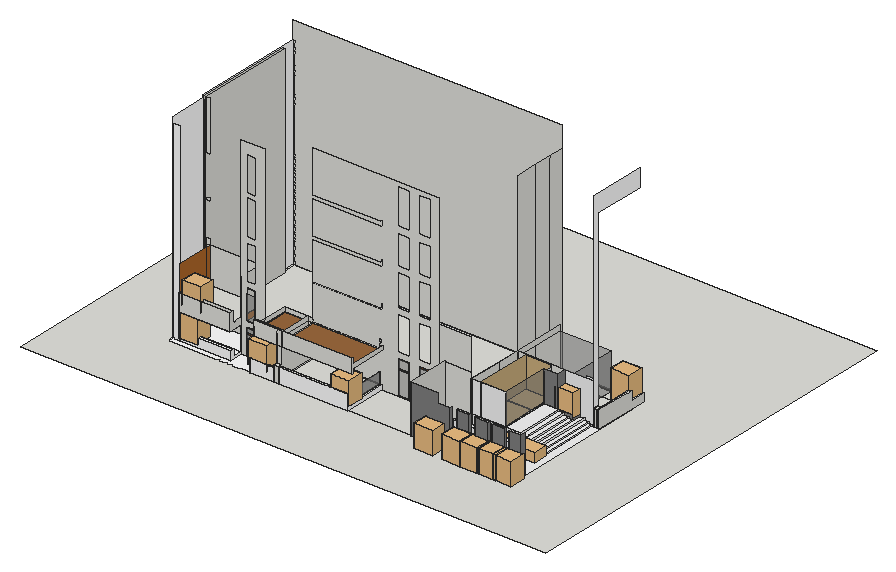
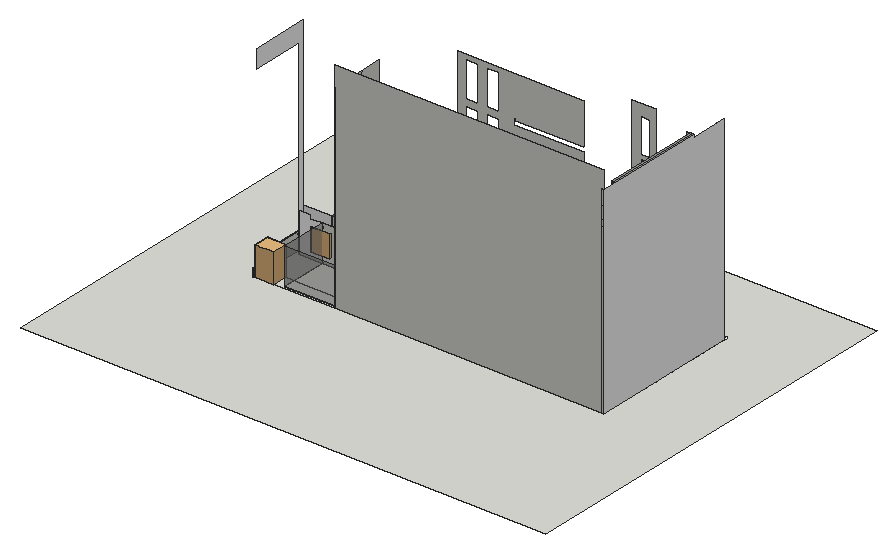
# SketchUp Ruby script. Lengths in inches.
U = 1.inch
M = Sketchup.active_model
def pt(a) = Geom::Point3d.new(a.map { |v| v * U })
def face(e, loops, mat)
  f = e.add_face(loops[0].map { |a| pt(a) })
  loops[1..].each { |l| e.add_face(l.map { |a| pt(a) }).erase! }
  f.material = f.back_material = mat if mat
  f
end
# faces: each face lists its corners as indices into pts; further lists are holes
def faces(e, pts, list, mat = nil) = list.each { |f| face(e, (f[0].is_a?(Array) ? f : [f]).map { |l| l.map { |i| pts[i] } }, mat) }
# xy, xz, yz: faces in a plane at the given z, y or x. An outline is a flat list of corners, or four numbers for a rectangle; further outlines are holes
def ring(l) = l.size == 4 ? [[l[0], l[1]], [l[2], l[1]], [l[2], l[3]], [l[0], l[3]]] : l.each_slice(2).to_a
def flat(e, list, mat, &to3) = list.each { |f| face(e, (f[0].is_a?(Array) ? f : [f]).map { |l| ring(l).map { |u, v| to3.(u, v) } }, mat) }
def xy(e, z, list, mat = nil) = flat(e, list, mat) { |x, y| [x, y, z] }
def xz(e, y, list, mat = nil) = flat(e, list, mat) { |x, z| [x, y, z] }
def yz(e, x, list, mat = nil) = flat(e, list, mat) { |y, z| [x, y, z] }
def lines(e, pts, list) = list.each { |a, b| e.add_line(pt(pts[a]), pt(pts[b])) }
# prism: a flat outline (further loops are holes) pulled along v
def prism(e, loops, v, mat = nil)
  f = face(e, loops, mat); d = Geom::Vector3d.new(v.map { |x| x * U })
  f.pushpull(f.normal.samedirection?(d) ? d.length : -d.length)
end
def box(e, o, s, mat = nil) = prism(e, [[o, [o[0] + s[0], o[1], o[2]], [o[0] + s[0], o[1] + s[1], o[2]], [o[0], o[1] + s[1], o[2]]]], [0, 0, s[2]], mat)
def at(x, y, z, deg = 0) = Geom::Transformation.translation(pt([x, y, z])) * Geom::Transformation.rotation(ORIGIN, Z_AXIS, deg.degrees)
def axes(o, x, y, z) = Geom::Transformation.new([*x, 0, *y, 0, *z, 0, *pt(o).to_a, 1])
def part(name) = M.definitions.add(name)
# library, detail: a bought-in or finely detailed component or shape, given as its bounding box
def library(name, o, s) = part(name).tap { |d| box(d.entities, o, s) }
def detail(e, o, s) = box(e.add_group.entities, o, s)
def put(e, d, t, mat = nil) = e.add_instance(d, t).tap { |i| i.material = mat if mat }
def group(e, t, mat = nil) = e.add_group.tap { |g| g.transformation = t; g.material = mat if mat }.entities
root = M.entities
M.materials.add("[0128_White]").color = [255, 255, 255]
M.materials.add("[0129_WhiteSmoke]").color = [245, 245, 245]
M.materials.add("[0133_Gray]").color = [128, 128, 128]
M.materials.add("[Translucent Glass Gray]").color = [128, 128, 128]
M.materials["[Translucent Glass Gray]"].alpha = 0.5
M.materials.add("[Wood Bamboo]").color = [177, 105, 43]
M.materials.add("[Wood Floor Light]").color = [204, 176, 127]
M.materials.add("[Wood Floor]").color = [155, 105, 61]
M.materials.add("[Wood Veneer 01]").color = [120, 70, 37]
c1 = library("Plant+(3)",[-15.5,2.64,0],[117.71,96.38,184.75])
c2 = library("car\#1",[0.01,0.03,0.02],[18.76,39.97,12.32])
xy(root,0,[[[0,0,2055.4375,1614.25],[326.88,313.35,1705.61,313.35,1705.61,863.91,1698.8,863.91,1698.8,922.42,1381.11,922.42,1381.11,909.71,1380.91,863.91,1380.91,922.03,328.44,922.03,328.44,863.91,326.88,863.91]],[740.81,313.35,740.81,480.63,648.14,480.63,648.14,384.82,555.3,384.82,555.3,480.63,341.11,480.63,341.11,863.91,334.36,863.91,334.36,922.03,1380.91,922.03,1380.91,863.91,1380.59,789.03,1380.23,703.91,1381.11,703.91,1381.11,480.63,760.05,480.63,760.05,313.35],[648.14,313.35,740.81,384.82],[760.05,313.35,1030.72,480.63],[1030.72,313.35,1277.17,480.63],
  [1277.17,313.35,1277.17,332.67,1705.61,332.67,1705.61,315.28,1659.15,315.28,1659.15,322.22,1429.5,322.22,1429.5,313.35],[1429.5,313.35,1429.5,322.22,1452.81,322.22,1452.81,315.91,1502.3,315.91,1502.3,322.22,1524.96,322.22,1524.96,313.35],[1524.96,313.35,1576.59,322.22],[1576.59,313.35,1576.59,322.22,1590.59,322.22,1590.59,315.41,1641.67,315.41,1641.67,322.22,1659.15,322.22,1659.15,315.28,1705.61,315.28,1705.61,313.35],[1590.59,315.41,1641.67,322.22],
  [1452.81,315.91,1502.3,322.22],[326.88,334.16,328.44,863.91],[328.44,334.16,334.36,922.03],[334.36,334.16,356.17,480.63],[648.14,384.82,740.81,480.63],
  [1381.11,389.82,1635.38,406.46],[334.36,480.63,341.11,863.91],[1381.11,480.63,1381.11,703.91,1567.08,703.91,1567.08,669.54,1512.23,669.54,1512.23,480.63],[1512.23,480.63,1549.17,611.07],[1549.17,480.63,1655.44,611.07],
  [1655.44,480.63,1672.48,611.07],[1512.23,611.07,1549.17,669.54],[1549.17,611.07,1549.17,669.54,1567.08,669.54,1567.08,703.91,1655.44,703.91,1655.44,611.07],[1655.44,611.07,1672.48,703.91],[1380.23,703.91,1380.59,789.03,1381.11,789.03,1381.11,703.91],
  [1381.11,703.91,1678.36,725.91],[1678.36,703.91,1678.36,725.91,1583.5,725.91,1583.5,863.91,1690.68,863.91,1690.68,703.91],[1690.68,703.91,1690.68,703.97,1698.8,703.97,1698.8,863.91,1705.61,863.91,1705.61,703.91],[1690.68,703.97,1698.8,863.91],[1381.11,725.91,1583.5,863.91],
  [1380.59,789.03,1380.91,863.91,1381.11,863.91,1381.11,789.03],[1380.91,863.91,1381.11,909.71,1381.11,863.91],[1381.11,863.91,1583.5,909.71],[1583.5,863.91,1583.5,909.71,1381.11,909.71,1381.11,922.42,1690.68,922.42,1690.68,863.91],[1690.68,863.91,1698.8,922.42]])
xy(root,0,[[326.88,313.35,334.36,334.16],[334.36,313.35,334.36,334.16,555.3,334.16,555.3,384.82,648.14,384.82,648.14,313.35],[356.17,384.82,555.3,480.63]],"[0128_White]")
xy(root,0,[[1277.17,332.67,1277.17,389.82,1635.38,389.82,1635.38,406.46,1381.11,406.46,1381.11,480.63,1672.48,480.63,1672.48,703.91,1705.61,703.91,1705.61,332.67]],"[0129_WhiteSmoke]")
xy(root,5.58,[[1659.15,480.63,1672.48,703.91]],"[0129_WhiteSmoke]")
xy(root,9.125,[[356.17,347.73,555.3,384.82]],"[0128_White]")
xy(root,11.51,[[1643.25,480.63,1659.15,703.91]],"[0129_WhiteSmoke]")
xy(root,14.6875,[[659.01,318.04,740.81,384.82]])
xy(root,15.875,[[760.05,319.99,1021.57,480.63],[1022.99,319.99,1030.72,480.63]])
xy(root,17.08,[[1625.72,480.63,1643.25,703.91]],"[0129_WhiteSmoke]")
xy(root,22.14,[[1551.96,669.54,1622.94,701.12]],"[0133_Gray]")
xy(root,22.7,[[1610.9,480.63,1625.72,666.75]],"[0129_WhiteSmoke]")
xy(root,26.58,[[1551.96,669.54,1567.08,701.12]])
xy(root,28.58,[[1591.2,480.63,1610.9,666.75]],"[0129_WhiteSmoke]")
xy(root,29,[[1690.68,862.91,1698.8,922.42]])
xy(root,33.0625,[[356.17,334.16,555.3,347.73]],"[0128_White]")
xy(root,33.7,[[1571.32,480.63,1591.2,666.75]],"[0129_WhiteSmoke]")
xy(root,38.58,[[1512.23,480.63,1571.32,669.54]],"[0129_WhiteSmoke]")
xy(root,38.58,[[1571.32,666.75,1571.32,669.54,1622.94,669.54,1622.94,701.12,1567.08,701.12,1567.08,703.91,1625.72,703.91,1625.72,666.75]],"[0133_Gray]")
xy(root,39.9375,[[1381.11,480.63,1512.23,611.07]])
xy(root,39.94,[[1381.11,611.07,1381.11,703.91,1512.23,703.91,1512.23,701.73,1414.17,701.73,1414.17,611.07]])
xy(root,39.94,[[1414.17,481.99,1512.23,611.07],[1414.17,611.07,1512.23,701.73]],"[Wood Floor Light]")
xy(root,50.0625,[[648.14,313.35,659.01,384.82],[659.01,313.35,740.81,318.04]])
xy(root,56.9375,[[1381.11,389.82,1635.38,406.46]],"[0129_WhiteSmoke]")
xy(root,60.3125,[[740.81,313.35,760.05,329.32],[760.05,313.35,1030.72,319.99],[1021.57,319.99,1022.99,480.63]])
xy(root,64.8125,[[1678.36,703.91,1690.68,725.91],[1690.68,703.97,1698.8,862.91]])
xy(root,103.72,[[341.11,480.48,356.17,480.63]])
xy(root,103.72,[[356.17,329.32,555.3,480.63]],"[Wood Bamboo]")
xy(root,121.02,[[648.14,329.32,760.05,334.07],[760.05,329.32,1031.24,333.65]])
xy(root,129.39,[[356.17,342.5,555.3,480.63],[341.11,480.44,356.17,480.63]])
xy(root,139.33,[[648.14,334.07,651.98,480.63]])
xy(root,139.33,[[760.05,333.65,1031.24,480.63],[651.98,334.07,740.81,480.63]],"[Wood Floor]")
xz(root,313.35,[[740.81,0,760.05,60.3125]])
xz(root,313.35,[[648.14,0,740.81,50.0625],[760.05,0,1030.72,60.3125]],"[0128_White]")
xz(root,313.35,[[1277.17,0,1429.5,0,1429.5,150.5625,1381.11,150.5625,1381.11,186.6875,1277.17,186.6875],[1524.96,0,1576.59,150.5625]],"[0133_Gray]")
xz(root,315.28,[[1659.15,0,1705.61,150.5625]],"[0133_Gray]")
xz(root,315.41,[[1590.59,0,1641.67,150.5625]],"[0133_Gray]")
xz(root,315.91,[[1452.81,0,1502.3,150.5625]],"[0133_Gray]")
xz(root,318.04,[[659.01,14.6875,740.81,50.0625]])
xz(root,319.99,[[760.05,15.875,1021.57,60.3125],[1022.99,15.875,1030.72,60.3125]])
xz(root,322.22,[[1452.81,0,1502.3,150.5625],[1524.96,0,1576.59,150.5625],[1590.59,0,1641.67,150.5625]])
xz(root,329.32,[[740.81,60.3125,760.05,121.02],[356.17,103.72,555.3,170.64],[648.14,121.02,740.81,178.02],[740.81,121.02,760.05,178.02],[760.05,121.02,1031.24,178.02]])
xz(root,333.65,[[760.05,121.02,1031.24,139.33]])
xz(root,334.07,[[648.14,121.02,648.14,139.33,740.81,139.33,740.81,155.59,648.14,155.59,648.14,178.02,760.05,178.02,760.05,121.02]])
xz(root,334.16,[[328.44,0,356.17,752.13],[356.17,0,555.3,33.0625]],"[0128_White]")
xz(root,342.5,[[356.17,129.39,555.3,170.64]])
xz(root,347.73,[[356.17,9.125,555.3,33.0625]],"[0128_White]")
xz(root,384.82,[[[555.3,0,575.9,0,575.9,103.89,612.02,103.89,612.02,0,648.14,0,648.14,751.9375,555.3,751.9375],[575.9,417.33,612.02,558.06],[575.9,261.04,612.02,397.85],[575.9,572.25,612.02,707],[575.9,121.02,612.02,242]],[648.14,0,740.81,0,740.81,14.6875,659.01,14.6875,659.01,50.0625,648.14,50.0625]])
xz(root,384.82,[[356.17,0,555.3,9.125]],"[0128_White]")
xz(root,384.82,[[578.59,2.6875,609.33,77.53],[578.59,83.51,609.33,101.2],[578.28,123.4,609.63,220.2]],"[Translucent Glass Gray]")
xz(root,384.82,[[575.9,0,612.02,0,612.02,103.89,575.9,103.89,575.9,83.51,578.59,83.51,578.59,101.2,609.33,101.2,609.33,2.6875,578.59,2.6875,578.59,77.53,575.9,77.53],[575.9,77.53,578.59,83.51],[578.59,77.53,609.33,83.51],[[575.9,121.02,612.02,242],[578.28,123.4,609.63,239.61]]],"[Wood Veneer 01]")
xz(root,389.82,[[1381.11,0,1635.38,56.9375]],"[0129_WhiteSmoke]")
xz(root,406.46,[[1381.11,0,1635.38,56.9375]])
xz(root,480.63,[[334.36,0,341.11,0,341.11,103.72,356.17,103.72,356.17,129.39,341.11,129.39,341.11,268.96,356.17,268.96,356.17,292.29,341.11,292.29,341.11,425.41,356.17,425.41,356.17,434.15,341.11,434.15,341.11,590.28,356.17,590.28,356.17,784.875,341.11,784.875,341.11,774.125,334.36,774.125],[341.11,0,356.17,103.72],[356.17,0,555.3,103.72],[648.14,0,740.81,139.33],[760.05,0,1030.72,0,1030.72,15.875,1022.99,15.875,1022.99,60.3125,1021.57,60.3125,1021.57,15.875,760.05,15.875],
  [[1030.72,0,1092.83,0,1092.83,133,1138.93,133,1138.93,0,1175.01,0,1175.01,133,1221,133,1221,0,1253.63,0,1253.63,752.13,760.05,752.13,760.05,588.63,1026.8,588.63,1026.8,625.94,1028.375,625.94,1028.375,595.76,1031.24,595.76,1031.24,572.25,760.05,572.25,760.05,444.84,1024.58,444.84,1024.58,478.66,1026.48,478.66,1026.48,455.53,1031.24,455.53,1031.24,429.57,760.05,429.57,760.05,284.41,1025.87,284.41,1025.87,326.04,1026.95,326.04,1026.95,302.85,1031.24,302.85,1031.24,278.66,760.05,278.66,760.05,142.65,1021.125,142.65,1021.125,178.02,1023.09,178.02,1023.09,155.59,1031.24,155.59,1031.24,139.33,760.05,139.33,760.05,15.875,1021.57,15.875,1021.57,60.3125,1022.99,60.3125,1022.99,15.875,1030.72,15.875],[1092.83,595.76,1138.93,734.94],[1175.01,595.76,1221,734.94],[1092.83,153.9375,1138.93,286.11],[1175.01,153.9375,1221,286.11],[1092.83,307.875,1138.93,433.75],[1175.01,307.875,1221,433.75],[1092.83,455.53,1138.93,570.34],[1175.01,455.53,1221,570.34]],[1253.63,0,1277.17,0,1277.17,186.6875,1281.11,186.6875,1281.11,214.5625,1281.7,214.5625,1281.7,186.6875,1378.67,186.6875,1378.67,307.875,1253.63,307.875],[1277.17,0,1277.17,186.6875,1281.11,186.6875,1281.11,214.5625,1281.7,214.5625,1281.7,186.6875,1378.67,186.6875,1378.67,0],[1378.67,0,1381.11,150.5625],[341.11,129.39,356.17,268.96],
  [356.17,129.39,555.3,268.96],[648.14,139.33,740.81,155.59],[740.81,139.33,1031.24,139.33,1031.24,155.59,1023.09,155.59,1023.09,178.02,1021.125,178.02,1021.125,142.65,760.05,142.65,760.05,155.59,740.81,155.59]])
xz(root,480.63,[[1381.11,0,1512.23,39.9375],[1512.23,0,1549.17,38.58],[1549.17,0,1549.17,38.58,1571.32,38.58,1571.32,33.7,1591.2,33.7,1591.2,28.58,1610.9,28.58,1610.9,22.7,1625.72,22.7,1625.72,17.08,1643.25,17.08,1643.25,11.51,1659.15,11.51,1659.15,5.58,1672.48,5.58,1672.48,0],[1381.11,39.9375,1512.23,161]],"[0129_WhiteSmoke]")
xz(root,480.63,[[1095.85,3.01,1135.91,92.59],[1178.3125,3.31,1217.69,93.86],[1095.85,97.125,1135.91,129.98],[1178.3125,98.55,1217.69,129.6875]],"[Translucent Glass Gray]")
xz(root,480.63,[[[1092.83,0,1138.93,133],[1095.85,3.01,1135.91,129.98]],[[1175.01,0,1221,133],[1178.3125,3.31,1217.69,129.6875]],[1095.85,92.59,1135.91,97.125],[1178.3125,93.86,1217.69,98.55]],"[Wood Veneer 01]")
xz(root,481.99,[[1414.17,39.94,1512.23,161]],"[Wood Floor Light]")
xz(root,611.07,[[1381.11,39.9375,1512.23,39.94]])
xz(root,666.75,[[1610.9,22.7,1610.9,28.58,1591.2,28.58,1591.2,33.7,1571.32,33.7,1571.32,38.58,1625.72,38.58,1625.72,22.7]],"[0133_Gray]")
xz(root,669.54,[[1512.23,0,1512.23,38.58,1567.08,38.58,1567.08,26.58,1551.96,26.58,1551.96,22.14,1567.08,22.14,1567.08,0],[1551.96,22.14,1567.08,26.58],[1567.08,22.14,1622.94,26.58]])
xz(root,669.54,[[1567.08,26.58,1622.94,38.58],[1512.23,38.58,1567.08,161]],"[0133_Gray]")
xz(root,701.12,[[1551.96,22.14,1622.94,26.58],[1567.08,26.58,1622.94,38.58]],"[0133_Gray]")
xz(root,701.73,[[1414.17,39.94,1512.23,161]],"[Wood Floor Light]")
xz(root,703.91,[[1380.23,0,1381.11,379.5625],[1381.11,0,1512.23,39.94],[1512.23,0,1567.08,161],[1567.08,0,1611.26,38.58],[1611.26,0,1611.26,38.58,1625.72,38.58,1625.72,17.08,1643.25,17.08,1643.25,11.51,1655.44,11.51,1655.44,0],
  [1655.44,0,1655.44,11.51,1659.15,11.51,1659.15,5.58,1672.48,5.58,1672.48,0],[1678.36,0,1690.68,64.8125],[1381.11,39.94,1512.23,161]])
xz(root,703.91,[[1672.48,0,1672.48,5.58,1659.15,5.58,1659.15,11.51,1643.25,11.51,1643.25,17.08,1625.72,17.08,1625.72,38.58,1567.08,38.58,1567.08,161,1678.36,161,1678.36,0]],"[0129_WhiteSmoke]")
xz(root,703.97,[[1690.68,0,1698.8,64.8125]],"[0128_White]")
xz(root,725.91,[[1381.11,0,1583.5,140.13]])
xz(root,725.91,[[1583.5,0,1678.36,0,1678.36,153.57,1632.4375,153.57,1632.4375,140.13,1583.5,140.13]],"[0128_White]")
xz(root,862.91,[[1690.68,29,1698.8,64.8125]])
xz(root,863.91,[[334.36,0,341.11,784.875]])
xz(root,909.71,[[1381.11,0,1583.5,141.5625]],"[Translucent Glass Gray]")
xz(root,922.03,[[328.44,0,334.36,784.875],[334.36,0,334.36,784.875,328.44,784.875,328.44,855,1378.67,855,1378.67,784.875,1380.91,784.875,1380.91,0]])
xz(root,922.42,[[1690.68,0,1698.8,29]])
yz(root,328.44,[[334.16,0,922.03,0,922.03,784.875,480.63,784.875,480.63,774.125,334.16,774.125]],"[0128_White]")
yz(root,334.36,[[480.63,0,863.91,784.875]])
yz(root,341.11,[[480.63,0,480.63,103.72,480.48,103.72,480.44,129.39,480.63,129.39,480.63,268.96,480.24,268.96,480.21,292.29,480.63,292.29,480.63,425.41,480.02,425.41,480.01,434.15,480.63,434.15,480.63,590.28,479.78,590.28,479.76,607.98,479.76,774.125,480.63,774.125,480.63,784.875,863.91,784.875,863.91,0]])
yz(root,356.17,[[480.63,0,480.48,103.72,480.63,103.72],[329.32,103.72,334.16,170.64],[334.16,103.72,334.16,170.64,342.5,170.64,342.5,129.39,480.44,129.39,480.48,103.72],[480.48,103.72,480.44,129.39,480.63,129.39,480.63,103.72],[480.44,129.39,480.24,268.96,480.63,268.96,480.63,129.39]])
yz(root,356.17,[[334.16,0,334.16,33.0625,347.73,33.0625,347.73,9.125,384.82,9.125,384.82,0]],"[0128_White]")
yz(root,356.17,[[384.82,0,384.82,9.125,347.73,9.125,347.73,33.0625,334.16,33.0625,334.16,103.72,480.48,103.72,480.63,0],[342.5,129.39,342.5,170.64,334.16,170.64,334.16,259.34,335.15,259.34,335.15,268.96,458.97,268.96,458.97,129.39],[458.97,129.39,458.97,268.96,480.24,268.96,480.44,129.39]],"[Wood Bamboo]")
yz(root,555.3,[[384.82,0,480.63,103.72],[329.32,103.72,384.82,103.72,384.82,129.39,342.5,129.39,342.5,170.64,329.32,170.64],[384.82,129.39,480.63,268.96]])
yz(root,555.3,[[334.16,0,334.16,33.0625,347.73,33.0625,347.73,9.125,384.82,9.125,384.82,0]],"[0128_White]")
yz(root,648.14,[[384.82,0,480.63,121.02],[329.32,121.02,334.07,139.33],[334.07,121.02,384.82,139.33],[384.82,121.02,480.63,139.33],[329.32,139.33,384.82,155.59],
  [384.82,139.33,480.63,155.59]])
yz(root,648.14,[[313.35,0,384.82,50.0625]],"[0128_White]")
yz(root,659.01,[[318.04,14.6875,384.82,50.0625]])
yz(root,740.81,[[313.35,0,313.35,50.0625,318.04,50.0625,318.04,14.6875,384.82,14.6875,384.82,0],[384.82,0,384.82,14.6875,318.04,14.6875,318.04,50.0625,313.35,50.0625,313.35,60.3125,329.32,60.3125,329.32,139.33,480.63,139.33,480.63,0],[329.32,139.33,334.07,155.59],[334.07,139.33,480.63,155.59]])
yz(root,760.05,[[313.35,0,480.63,0,480.63,15.875,319.99,15.875,319.99,60.3125,313.35,60.3125],[319.99,15.875,480.63,15.875,480.63,139.33,334.07,139.33,334.07,121.02,329.32,121.02,329.32,60.3125,319.99,60.3125],[329.32,121.02,333.65,121.02,333.65,139.33,334.07,139.33,334.07,178.02,329.32,178.02],[333.65,121.02,334.07,139.33],[333.65,121.02,334.07,139.33]])
yz(root,1021.57,[[319.99,15.875,480.63,60.3125]],"[Translucent Glass Gray]")
yz(root,1022.99,[[319.99,15.875,480.63,60.3125]],"[Translucent Glass Gray]")
yz(root,1030.72,[[313.35,0,313.35,60.3125,319.99,60.3125,319.99,15.875,480.63,15.875,480.63,0]],"[0128_White]")
yz(root,1031.24,[[329.32,121.02,333.65,121.02,333.65,139.33,480.63,139.33,480.63,155.59,334.2,155.59,334.2,178.02,329.32,178.02]])
yz(root,1277.17,[[313.35,0,480.63,186.6875]])
yz(root,1380.91,[[863.91,0,922.03,774.125]])
yz(root,1381.11,[[389.82,0,406.46,56.9375],[480.63,0,611.07,39.9375],[611.07,0,703.91,39.94],[703.91,0,725.91,0,725.91,141.5625,909.71,141.5625,909.71,161,703.91,161],[725.91,0,789.03,140.13],
  [789.03,0,909.71,140.13],[480.63,39.9375,611.07,161],[611.07,39.94,703.91,161]])
yz(root,1414.17,[[481.99,39.94,701.73,161]],"[Wood Floor Light]")
yz(root,1429.5,[[313.35,0,322.22,150.5625]],"[0133_Gray]")
yz(root,1452.81,[[315.91,0,322.22,150.5625]])
yz(root,1502.3,[[315.91,0,322.22,150.5625]],"[0133_Gray]")
yz(root,1512.23,[[480.63,0,611.07,38.58],[611.07,0,669.54,38.58],[480.63,38.58,611.07,39.9375],[611.07,38.58,668.18,39.94],[668.18,38.58,669.54,39.94],
  [480.63,39.9375,480.63,146.92,481.99,146.92,481.99,39.94,611.07,39.94,611.07,39.9375],[669.54,39.94,701.73,148.28],[701.73,39.94,703.91,161]])
yz(root,1512.23,[[481.99,39.94,669.54,161]],"[Translucent Glass Gray]")
yz(root,1524.96,[[313.35,0,322.22,150.5625]])
yz(root,1551.96,[[669.54,22.14,701.12,26.58]])
yz(root,1567.08,[[669.54,26.58,669.54,161,703.91,161,703.91,38.58,701.12,38.58,701.12,26.58]],"[0133_Gray]")
yz(root,1571.32,[[480.63,33.7,666.75,38.58]],"[0129_WhiteSmoke]")
yz(root,1576.59,[[313.35,0,322.22,150.5625]],"[0133_Gray]")
yz(root,1583.5,[[725.91,0,909.71,141.5625]],"[Translucent Glass Gray]")
yz(root,1590.59,[[315.41,0,322.22,150.5625]])
yz(root,1591.2,[[480.63,28.58,666.75,33.7]],"[0129_WhiteSmoke]")
yz(root,1610.9,[[480.63,22.7,666.75,28.58]],"[0129_WhiteSmoke]")
yz(root,1622.94,[[669.54,22.14,701.12,26.58],[669.54,26.58,701.12,38.58]])
yz(root,1625.72,[[480.63,17.08,666.75,22.7]],"[0129_WhiteSmoke]")
yz(root,1625.72,[[666.75,17.08,703.91,38.58]],"[0133_Gray]")
yz(root,1635.38,[[389.82,0,406.46,56.9375]],"[0129_WhiteSmoke]")
yz(root,1641.67,[[315.41,0,322.22,150.5625]],"[0133_Gray]")
yz(root,1643.25,[[480.63,11.51,703.91,17.08]],"[0129_WhiteSmoke]")
yz(root,1659.15,[[315.28,0,322.22,150.5625]])
yz(root,1659.15,[[480.63,5.58,703.91,11.51]],"[0129_WhiteSmoke]")
yz(root,1672.48,[[480.63,0,703.91,5.58]],"[0129_WhiteSmoke]")
yz(root,1678.36,[[703.91,0,725.91,64.8125]])
yz(root,1678.36,[[703.91,64.8125,703.91,808.62,929.53,808.62,929.53,738.98,725.91,738.98,725.91,64.8125]],"[0128_White]")
yz(root,1690.68,[[703.91,0,703.97,64.8125],[703.97,0,703.97,64.8125,862.91,64.8125,862.91,29,922.42,29,922.42,0]])
yz(root,1698.8,[[703.97,0,922.42,0,922.42,29,862.91,29,862.91,64.8125,703.97,64.8125]])
yz(root,1705.61,[[315.28,0,332.67,150.5625]],"[0133_Gray]")
p = [[1380.59,789.03,0],[1380.59,789.03,774.125],[1380.23,703.91,774.125],[1380.23,703.91,651.9375],[1380.23,703.91,379.5625],[1380.23,703.91,0],
  [1380.91,863.91,0],[1380.91,863.91,774.125],[1378.67,480.63,161],[1381.11,703.91,161],[1381.11,703.91,39.94],[1378.67,480.63,39.94],
  [1378.67,480.63,150.5625],[356.17,480.48,103.72],[356.17,480.44,129.39],[341.11,480.44,129.39],[341.11,480.48,103.72],[651.98,334.07,139.33],
  [651.98,329.32,139.33]]
faces(root,p,[[0,1,2,3,4,5],[6,7,1,0],[8,9,10,11,12],[13,14,15,16]])
lines(root,p,[[17,18]])
put(root,c1,axes([1651.28,254.02,0],[0.62,0,0],[0,0.62,0],[0,0,0.4774]))
put(root,c1,axes([1343.03,254.02,0],[0.62,0,0],[0,0.62,0],[0,0,0.4774]))
put(root,c1,axes([1451.9,254.02,0],[0.62,0,0],[0,0.62,0],[0,0,0.4774]))
put(root,c1,axes([1523.03,254.02,0],[0.62,0,0],[0,0.62,0],[0,0,0.4774]))
put(root,c1,axes([1590.4,254.02,0],[0.62,0,0],[0,0.62,0],[0,0,0.4774]))
put(root,c1,axes([1627.3125,861.03,0],[0.62,0,0],[0,0.62,0],[0,0,0.62]))
put(root,c2,axes([1679.38,414.21,-0.05],[0,3.0284,0],[-3.63408,0,0],[0,0,3.0284]))
put(root,c1,axes([361.76,332.52,9.375],[0.62,0,0],[0,0.62,0],[0,0,0.4774]))
put(root,c1,axes([970.875,313.35,17.22],[0.62,0,0],[0,0.62,0],[0,0,0.4774]))
put(root,c1,axes([648.14,313.35,25.03],[0.62,0,0],[0,0.62,0],[0,0,0.4774]))
put(root,c1,axes([1562.375,667.91,26.58],[0.62,0,0],[0,0.62,0],[0,0,0.4774]))
put(root,c1,axes([378.02,329.32,129.39],[0.62,0,0],[0,0.62,0],[0,0,0.4774]))
